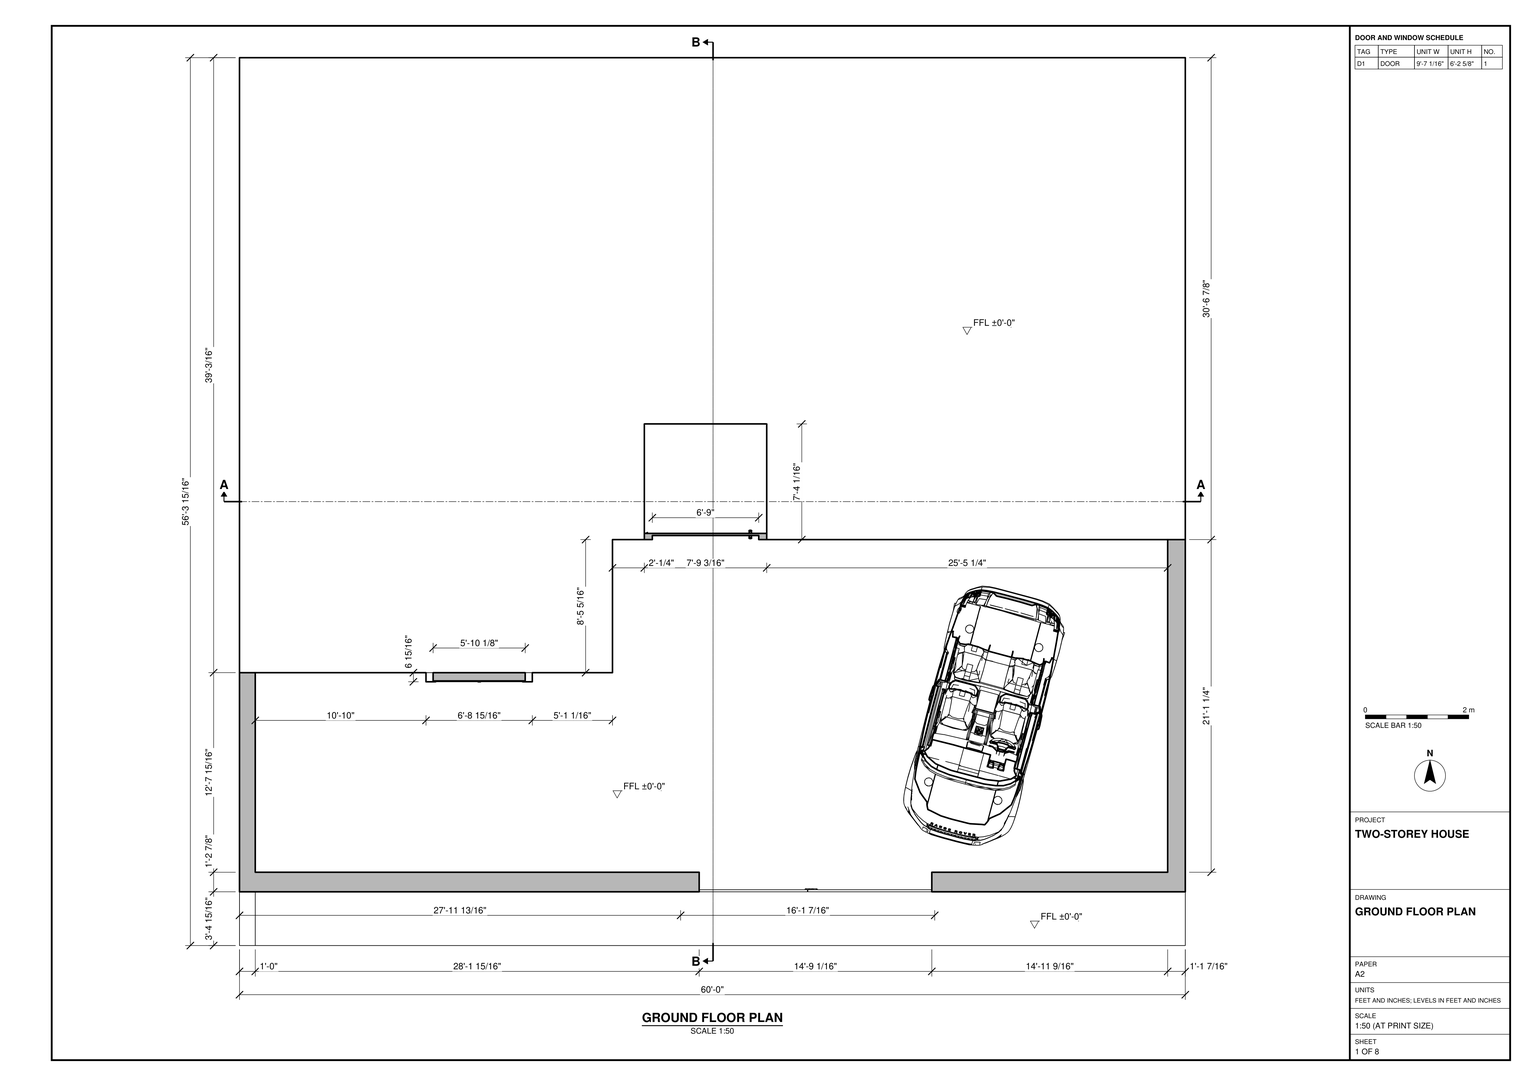
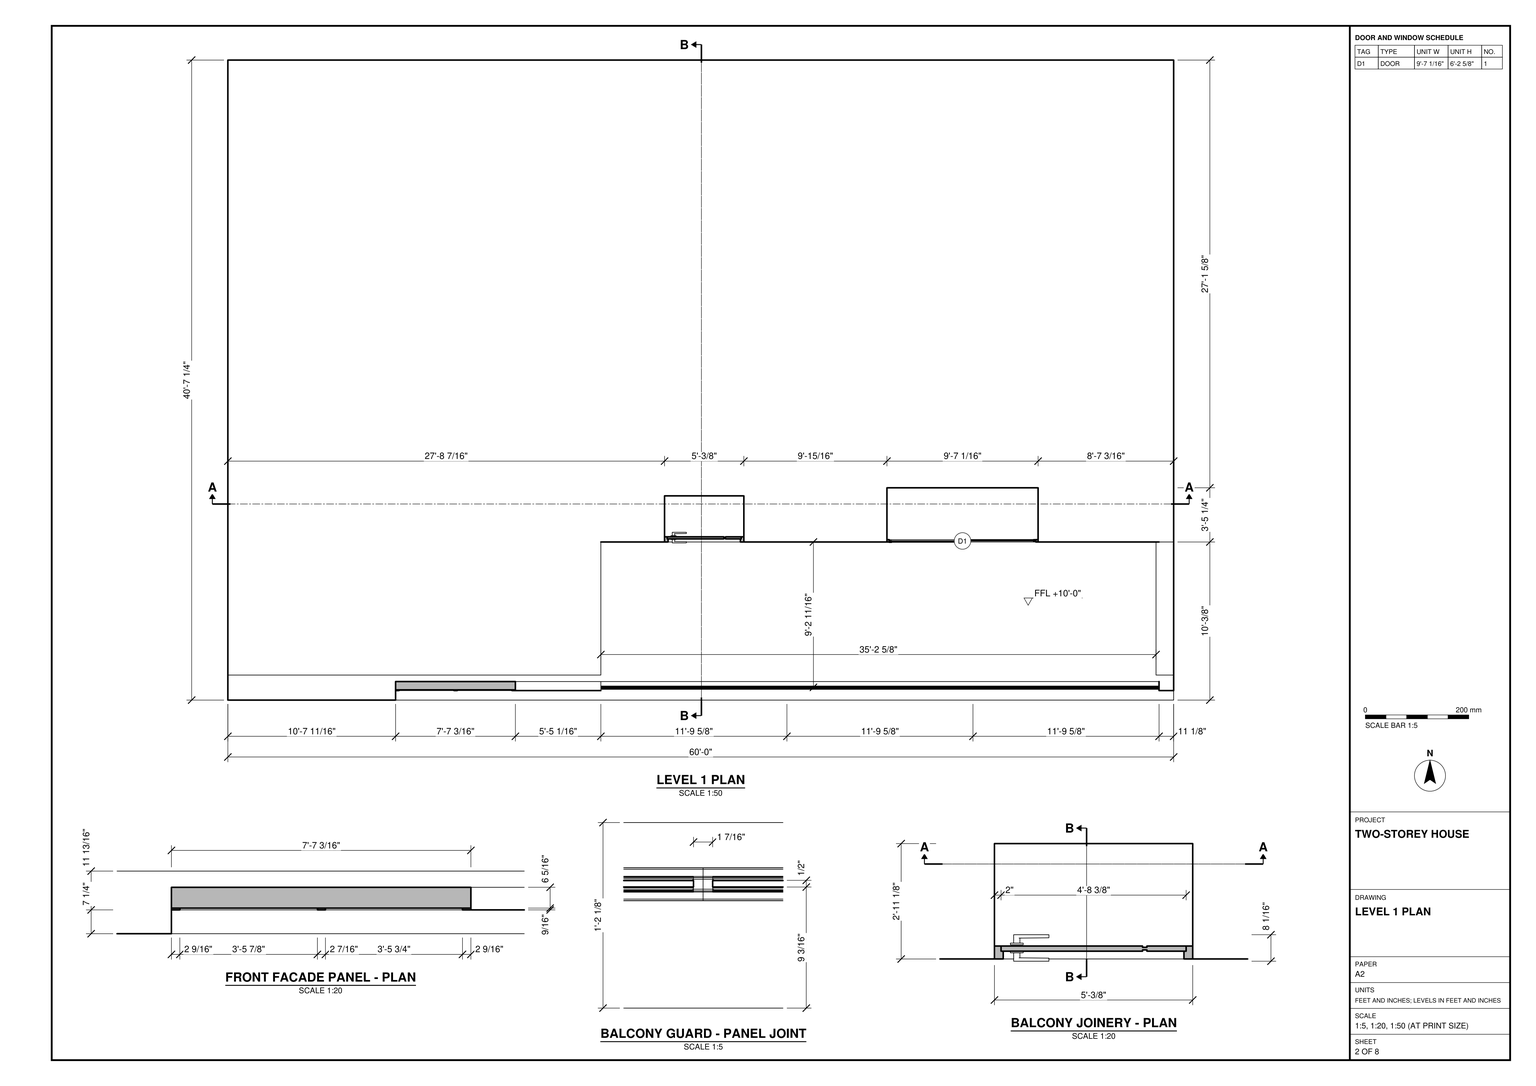
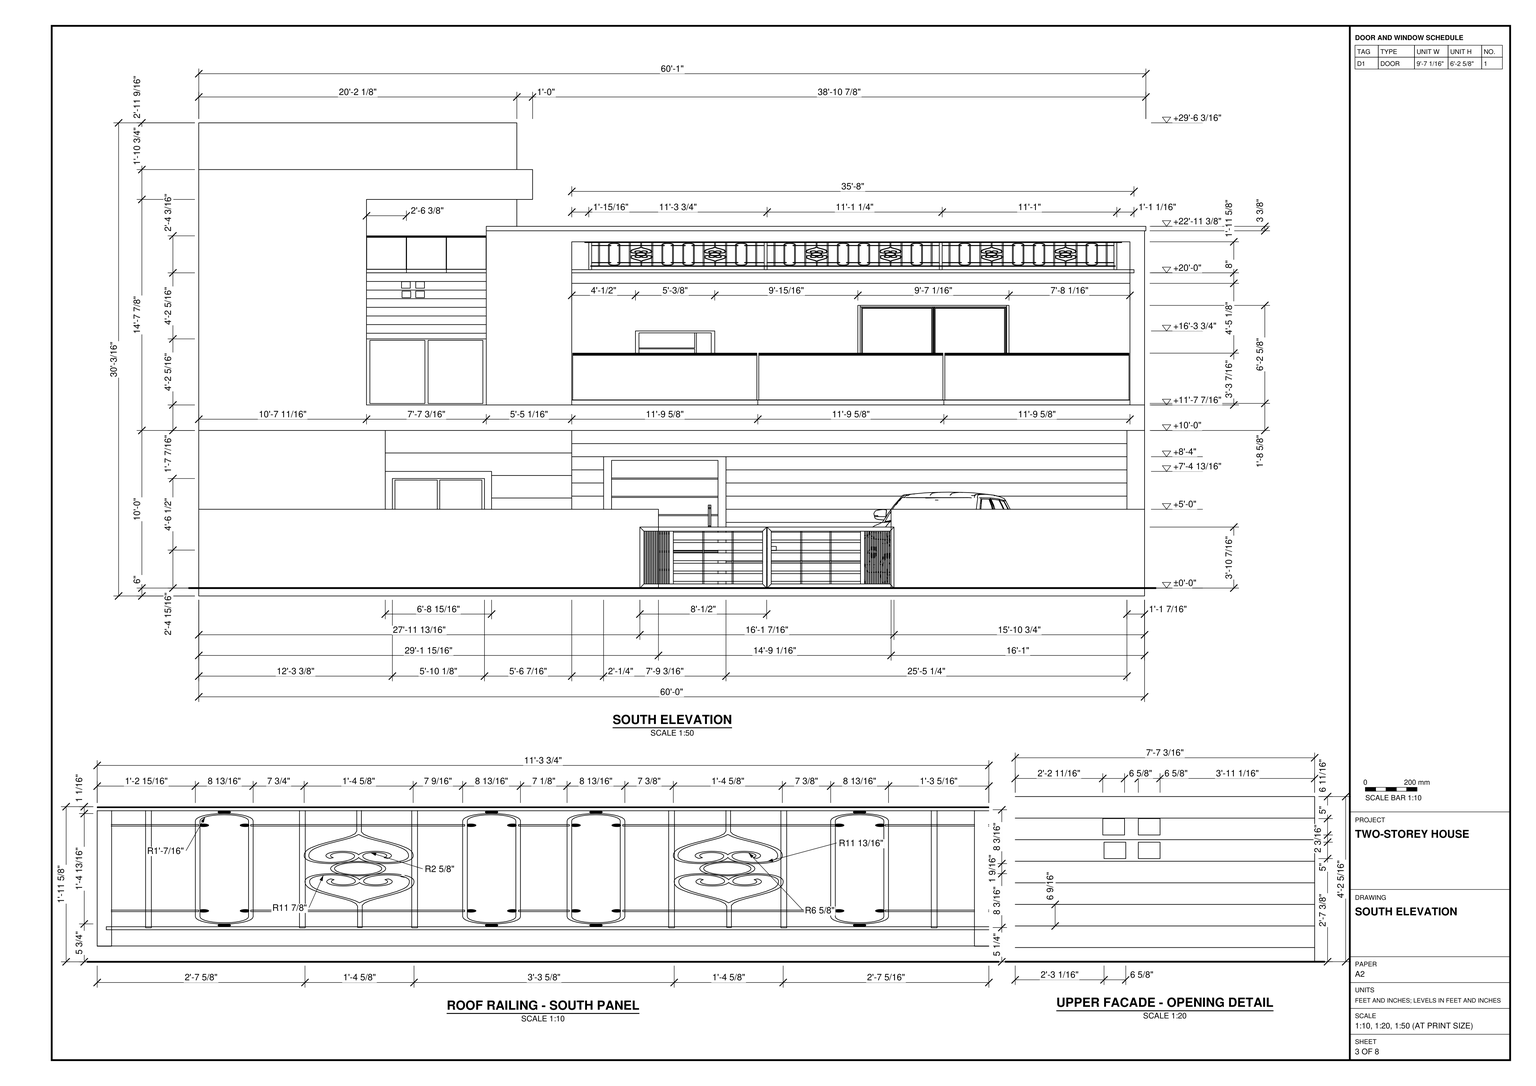
Build the two-storey house in SketchUp from task_files/diagram_01.pdf. Work in feet and inches. The overall model extents are 60'-1" along X, 56'-3 15/16" along Y and 30'-3/16" along Z. Set the ground floor at ±0'-0" and the upper floor at +10'-0".

Use the plans to place the stepped south wall: the left part projects into the forecourt, while the right part is set back behind the parking area. Model the floor slabs, exterior walls and low forecourt walls at the thicknesses drawn. Fit the double-leaf gate in the front wall and place the car on the right side of the forecourt.

Use the south elevation to set out the taller left volume, the flat roof slabs and the rectangular frame around the recessed upper balcony. Model the panel joints in the balcony guard, the wide door and the narrower joinery to its left. Follow the details for the banded facade panel and the repeating railing along the roof. Decor and loose items may be represented by any suitable library component.

Keep the walls, slabs and roof separate as groups or components, and group each furniture or joinery piece separately. Use components for repeated parts. Save one SketchUp model as output_files/two_storey_house_gated_forecourt_and_recessed_balcony.skp.

# SketchUp Ruby script. Lengths in inches.
U = 1.inch
M = Sketchup.active_model
def pt(a) = Geom::Point3d.new(a.map { |v| v * U })
def face(e, loops, mat)
  f = e.add_face(loops[0].map { |a| pt(a) })
  loops[1..].each { |l| e.add_face(l.map { |a| pt(a) }).erase! }
  f.material = f.back_material = mat if mat
  f
end
# faces: each face lists its corners as indices into pts; further lists are holes
def faces(e, pts, list, mat = nil) = list.each { |f| face(e, (f[0].is_a?(Array) ? f : [f]).map { |l| l.map { |i| pts[i] } }, mat) }
# xy, xz, yz: faces in a plane at the given z, y or x. An outline is a flat list of corners, or four numbers for a rectangle; further outlines are holes
def ring(l) = l.size == 4 ? [[l[0], l[1]], [l[2], l[1]], [l[2], l[3]], [l[0], l[3]]] : l.each_slice(2).to_a
def flat(e, list, mat, &to3) = list.each { |f| face(e, (f[0].is_a?(Array) ? f : [f]).map { |l| ring(l).map { |u, v| to3.(u, v) } }, mat) }
def xy(e, z, list, mat = nil) = flat(e, list, mat) { |x, y| [x, y, z] }
def xz(e, y, list, mat = nil) = flat(e, list, mat) { |x, z| [x, y, z] }
def yz(e, x, list, mat = nil) = flat(e, list, mat) { |y, z| [x, y, z] }
def lines(e, pts, list) = list.each { |a, b| e.add_line(pt(pts[a]), pt(pts[b])) }
# prism: a flat outline (further loops are holes) pulled along v
def prism(e, loops, v, mat = nil)
  f = face(e, loops, mat); d = Geom::Vector3d.new(v.map { |x| x * U })
  f.pushpull(f.normal.samedirection?(d) ? d.length : -d.length)
end
def box(e, o, s, mat = nil) = prism(e, [[o, [o[0] + s[0], o[1], o[2]], [o[0] + s[0], o[1] + s[1], o[2]], [o[0], o[1] + s[1], o[2]]]], [0, 0, s[2]], mat)
def at(x, y, z, deg = 0) = Geom::Transformation.translation(pt([x, y, z])) * Geom::Transformation.rotation(ORIGIN, Z_AXIS, deg.degrees)
def axes(o, x, y, z) = Geom::Transformation.new([*x, 0, *y, 0, *z, 0, *pt(o).to_a, 1])
def part(name) = M.definitions.add(name)
# library, detail: a bought-in or finely detailed component or shape, given as its bounding box
def library(name, o, s) = part(name).tap { |d| box(d.entities, o, s) }
def detail(e, o, s) = box(e.add_group.entities, o, s)
def put(e, d, t, mat = nil) = e.add_instance(d, t).tap { |i| i.material = mat if mat }
def group(e, t, mat = nil) = e.add_group.tap { |g| g.transformation = t; g.material = mat if mat }.entities
root = M.entities
M.materials.add("2 ").color = [128, 128, 128]
M.materials["2 "].alpha = 0.5
M.materials.add("Glass_Tinted_Gray").color = [0, 0, 0]
M.materials["Glass_Tinted_Gray"].alpha = 0.125
M.materials.add("Material60").color = [234, 198, 157]
M.materials.add("RDFGXVY 1").color = [35, 53, 69]
M.materials.add("[0086_MediumAquamarine]").color = [16, 35, 30]
M.materials.add("[0135_DarkGray]").color = [81, 81, 81]
M.materials.add("[0137_Black]").color = [0, 0, 0]
M.materials.add("[Color M00]").color = [255, 255, 255]
M.materials.add("[Color M04]").color = [142, 142, 142]
M.materials.add("[Mirror 02]").color = [229, 229, 229]
M.materials.add("[Slate Light Tile]").color = [54, 54, 54]
M.materials.add("[Terrazzo Light Blue]").color = [196, 214, 227]
M.materials.add("[Wood Veneer 01]").color = [120, 70, 37]
M.materials.add("[Wood Veneer 01]1").color = [119, 70, 35]
M.materials.add("ertg dfy 1").color = [92, 92, 92]
c1 = library("Glass Railings(black Handrails)",[-57.04,-132.55,0],[169.29,2.52,28.17])
c2 = part("Box01")
box(c2.entities,[-226.9,-4,10.92],[453.97,2,2],"RDFGXVY 1")
c3 = part("Box33")
box(c3.entities,[-243.2,-14.58,-10.36],[486.37,14.58,10.5],"ertg dfy 1")
c4 = part("Box45")
box(c4.entities,[-155.57,-3.5,79.72],[8.78,1,1],"RDFGXVY 1")
c5 = part("Box46")
box(c5.entities,[-201.91,-3.5,79.72],[37.02,1,1],"RDFGXVY 1")
c6 = part("Box48")
box(c6.entities,[-226.6,-3.5,79.72],[15.69,1,1],"RDFGXVY 1")
c7 = part("Box50")
box(c7.entities,[-220.1,-3.75,12.2],[1,1.5,78.43],"RDFGXVY 1")
c8 = part("Box51")
box(c8.entities,[-228.47,-4.25,0],[2.5,2.5,90.63],"RDFGXVY 1")
c9 = part("Donut06")
prism(c9.entities,[[[-187.98,-2.25,52.57],[-187.62,-2.25,53.58],[-187.05,-2.25,54.47],[-186.3125,-2.25,55.21],[-185.43,-2.25,55.77],[-184.42,-2.25,56.13],[-183.32,-2.25,56.26],[-182.23,-2.25,56.13],[-181.22,-2.25,55.77],[-180.34,-2.25,55.21],[-179.59,-2.25,54.47],[-179.03,-2.25,53.58],[-178.67,-2.25,52.57],[-178.54,-2.25,51.48],[-178.67,-2.25,50.38],[-179.03,-2.25,49.38],[-179.59,-2.25,48.49],[-180.34,-2.25,47.75],[-181.22,-2.25,47.18],[-182.23,-2.25,46.82],[-183.32,-2.25,46.7],[-184.42,-2.25,46.82],[-185.43,-2.25,47.18],[-186.3125,-2.25,47.75],[-187.05,-2.25,48.49],[-187.62,-2.25,49.38],[-187.98,-2.25,50.38],[-188.1,-2.25,51.48]],[[-186.52,-2.25,54.04],[-187.01,-2.25,53.28],[-187.32,-2.25,52.42],[-187.42,-2.25,51.48],[-187.32,-2.25,50.54],[-187.01,-2.25,49.68],[-186.52,-2.25,48.92],[-185.89,-2.25,48.28],[-185.125,-2.25,47.8],[-184.26,-2.25,47.49],[-183.32,-2.25,47.38],[-182.39,-2.25,47.49],[-181.52,-2.25,47.8],[-180.76,-2.25,48.28],[-180.125,-2.25,48.92],[-179.64,-2.25,49.68],[-179.33,-2.25,50.54],[-179.23,-2.25,51.48],[-179.33,-2.25,52.42],[-179.64,-2.25,53.28],[-180.125,-2.25,54.04],[-180.76,-2.25,54.68],[-181.52,-2.25,55.16],[-182.39,-2.25,55.47],[-183.32,-2.25,55.58],[-184.26,-2.25,55.47],[-185.125,-2.25,55.16],[-185.89,-2.25,54.68]]],[0,-1.5,0],"RDFGXVY 1")
c10 = library("Rectangl19",[-192.66,-3.75,54.81],[18.86,1.5,35.73])
c11 = part("Rectangl21")
prism(c11.entities,[[[-211.36,-2.25,18.49],[-211.49,-2.25,19.59],[-211.49,-2.25,83.23],[-211.36,-2.25,84.33],[-211,-2.25,85.34],[-210.43,-2.25,86.23],[-209.6875,-2.25,86.97],[-208.8,-2.25,87.54],[-207.79,-2.25,87.9],[-206.6875,-2.25,88.03],[-206.29,-2.25,88.03],[-205.1875,-2.25,87.9],[-204.18,-2.25,87.54],[-203.29,-2.25,86.97],[-202.54,-2.25,86.23],[-201.98,-2.25,85.34],[-201.62,-2.25,84.33],[-201.49,-2.25,83.23],[-201.49,-2.25,19.59],[-201.62,-2.25,18.49],[-201.98,-2.25,17.48],[-202.54,-2.25,16.59],[-203.29,-2.25,15.84],[-204.18,-2.25,15.28],[-205.1875,-2.25,14.92],[-206.29,-2.25,14.79],[-206.6875,-2.25,14.79],[-207.79,-2.25,14.92],[-208.8,-2.25,15.28],[-209.6875,-2.25,15.84],[-210.43,-2.25,16.59],[-211,-2.25,17.48]],[[-210.6875,-2.25,83.22],[-210.6875,-2.25,19.59],[-210.58,-2.25,18.68],[-210.28,-2.25,17.83],[-209.81,-2.25,17.09],[-209.1875,-2.25,16.47],[-208.44,-2.25,16],[-207.6,-2.25,15.7],[-206.68,-2.25,15.59],[-206.29,-2.25,15.59],[-205.375,-2.25,15.7],[-204.53,-2.25,16],[-203.79,-2.25,16.47],[-203.17,-2.25,17.09],[-202.7,-2.25,17.83],[-202.39,-2.25,18.68],[-202.29,-2.25,19.59],[-202.29,-2.25,83.22],[-202.39,-2.25,84.14],[-202.7,-2.25,84.98],[-203.17,-2.25,85.73],[-203.79,-2.25,86.35],[-204.53,-2.25,86.82],[-205.375,-2.25,87.12],[-206.29,-2.25,87.23],[-206.68,-2.25,87.23],[-207.6,-2.25,87.12],[-208.44,-2.25,86.82],[-209.1875,-2.25,86.35],[-209.81,-2.25,85.73],[-210.28,-2.25,84.98],[-210.58,-2.25,84.14]]],[0,-1.5,0],"RDFGXVY 1")
c12 = part("Rectangle0")
prism(c12.entities,[[[-231.96,-3.14,92.61],[-231.96,-1.96,92.53],[-231.96,-0.8125,92.24],[-231.96,0,91.89],[-231.96,0,89.89],[-231.96,-6,89.89],[-231.96,-6,91.89],[-231.96,-5.46,92.14],[-231.96,-4.32,92.48]]],[464.5,0,0],"RDFGXVY 1")
c13 = library("Sphere59",[-210.98,-3.9,79.34],[1.8,1.8,1.8])
c14 = library("Sphere66",[-207.6,-4.11,87.84],[2.22,2.22,2.22])
c15 = part("skp249")
put(c15.entities,c2,at(0,0,0))
put(c15.entities,c3,at(0,0,0))
put(c15.entities,c4,at(0,0,0))
put(c15.entities,c5,at(0,0,0))
put(c15.entities,c6,at(0,0,0))
put(c15.entities,c7,at(0,0,0))
put(c15.entities,c8,at(0,0,0))
put(c15.entities,c9,at(0,0,0))
put(c15.entities,c10,at(0,0,0))
put(c15.entities,c11,at(0,0,0))
put(c15.entities,c12,at(0,0,0))
put(c15.entities,c13,at(0,0,0))
put(c15.entities,c14,at(0,0,0))
put(c15.entities,c13,at(7.24,0,0))
put(c15.entities,c13,at(0,0,-56.78))
put(c15.entities,c13,at(7.24,0,-56.78))
put(c15.entities,c14,at(0,0,-75.08))
put(c15.entities,c6,at(0,0,-56.78))
put(c15.entities,c10,axes([0.14,0,102.9375],[1,0,0],[0,1,0],[0,0,-1]))
put(c15.entities,c5,at(0,0,-56.78))
put(c15.entities,c7,at(26.625,0,0))
put(c15.entities,c7,at(46.05,0,0))
put(c15.entities,c4,at(0,0,-56.78))
put(c15.entities,c14,at(46.25,0,0))
put(c15.entities,c13,at(46.25,0,0))
put(c15.entities,c13,at(53.48,0,0))
put(c15.entities,c13,at(53.48,0,-56.78))
put(c15.entities,c13,at(46.25,0,-56.78))
put(c15.entities,c14,at(46.25,0,-75.08))
put(c15.entities,c11,at(46.25,0,0))
put(c15.entities,c5,at(64.37,0,0))
put(c15.entities,c5,at(64.37,0,-56.78))
put(c15.entities,c11,at(64.3125,0,0))
put(c15.entities,c14,at(64.3125,0,-75.08))
put(c15.entities,c13,at(64.3125,0,-56.78))
put(c15.entities,c13,at(71.55,0,-56.78))
put(c15.entities,c13,at(71.55,0,0))
put(c15.entities,c13,at(64.3125,0,0))
put(c15.entities,c14,at(64.3125,0,0))
put(c15.entities,c7,at(90.5,0,0))
put(c15.entities,c7,at(109.92,0,0))
put(c15.entities,c10,at(63.875,0,0))
put(c15.entities,c10,axes([64.02,0,102.9375],[1,0,0],[0,1,0],[0,0,-1]))
put(c15.entities,c9,at(63.875,0,0))
put(c15.entities,c14,at(109.92,0,-75.08))
put(c15.entities,c13,at(117.16,0,0))
put(c15.entities,c13,at(109.92,0,0))
put(c15.entities,c14,at(109.92,0,0))
put(c15.entities,c13,at(109.92,0,-56.78))
put(c15.entities,c13,at(117.16,0,-56.78))
put(c15.entities,c11,at(109.92,0,0))
put(c15.entities,c7,at(135.9375,0,0))
put(c15.entities,c6,at(134.46,0,0))
put(c15.entities,c6,at(134.46,0,-56.78))
put(c15.entities,c8,at(151.78,0,0))
put(c15.entities,c7,at(151.78,0,0))
put(c15.entities,c6,at(151.78,0,0))
put(c15.entities,c6,at(151.78,0,-56.78))
put(c15.entities,c5,at(151.78,0,-56.78))
put(c15.entities,c7,at(178.4,0,0))
put(c15.entities,c7,at(197.83,0,0))
put(c15.entities,c14,at(151.78,0,-75.08))
put(c15.entities,c13,at(151.78,0,0))
put(c15.entities,c14,at(151.78,0,0))
put(c15.entities,c13,at(151.78,0,-56.78))
put(c15.entities,c13,at(159.01,0,-56.78))
put(c15.entities,c11,at(151.78,0,0))
put(c15.entities,c13,at(159.01,0,0))
put(c15.entities,c10,at(151.78,0,0))
put(c15.entities,c10,axes([151.92,0,102.9375],[1,0,0],[0,1,0],[0,0,-1]))
put(c15.entities,c9,at(151.78,0,0))
put(c15.entities,c5,at(151.78,0,0))
put(c15.entities,c4,at(151.78,0,0))
put(c15.entities,c4,at(151.78,0,-56.78))
put(c15.entities,c13,at(198.02,0,0))
put(c15.entities,c14,at(198.02,0,0))
put(c15.entities,c13,at(205.26,0,-56.78))
put(c15.entities,c11,at(198.02,0,0))
put(c15.entities,c13,at(205.26,0,0))
put(c15.entities,c13,at(198.02,0,-56.78))
put(c15.entities,c14,at(198.02,0,-75.08))
put(c15.entities,c5,at(216.14,0,0))
put(c15.entities,c5,at(216.14,0,-56.78))
put(c15.entities,c7,at(242.28,0,0))
put(c15.entities,c13,at(216.09,0,-56.78))
put(c15.entities,c14,at(216.09,0,-75.08))
put(c15.entities,c13,at(223.32,0,0))
put(c15.entities,c13,at(223.32,0,-56.78))
put(c15.entities,c14,at(216.09,0,0))
put(c15.entities,c11,at(216.09,0,0))
put(c15.entities,c13,at(216.09,0,0))
put(c15.entities,c7,at(261.69,0,0))
put(c15.entities,c10,at(215.65,0,0))
put(c15.entities,c10,axes([215.79,0,102.9375],[1,0,0],[0,1,0],[0,0,-1]))
put(c15.entities,c9,at(215.65,0,0))
put(c15.entities,c6,at(286.24,0,0))
put(c15.entities,c7,at(287.71,0,0))
put(c15.entities,c6,at(286.24,0,-56.78))
put(c15.entities,c7,at(303.21,0,0))
put(c15.entities,c13,at(268.93,0,0))
put(c15.entities,c14,at(261.69,0,-75.08))
put(c15.entities,c14,at(261.69,0,0))
put(c15.entities,c13,at(261.69,0,-56.78))
put(c15.entities,c13,at(268.93,0,-56.78))
put(c15.entities,c11,at(261.69,0,0))
put(c15.entities,c13,at(261.69,0,0))
put(c15.entities,c8,at(303.21,0,0))
put(c15.entities,c6,at(303.21,0,0))
put(c15.entities,c6,at(303.21,0,-56.78))
put(c15.entities,c7,at(329.83,0,0))
put(c15.entities,c7,at(349.26,0,0))
put(c15.entities,c5,at(303.21,0,0))
put(c15.entities,c5,at(303.21,0,-56.78))
put(c15.entities,c13,at(303.21,0,0))
put(c15.entities,c13,at(310.44,0,-56.78))
put(c15.entities,c14,at(303.21,0,-75.08))
put(c15.entities,c11,at(303.21,0,0))
put(c15.entities,c14,at(303.21,0,0))
put(c15.entities,c13,at(310.44,0,0))
put(c15.entities,c13,at(303.21,0,-56.78))
put(c15.entities,c10,at(303.21,0,0))
put(c15.entities,c9,at(303.21,0,0))
put(c15.entities,c10,axes([303.35,0,102.9375],[1,0,0],[0,1,0],[0,0,-1]))
put(c15.entities,c4,at(303.21,0,0))
put(c15.entities,c4,at(303.21,0,-56.78))
put(c15.entities,c14,at(349.45,0,0))
put(c15.entities,c13,at(349.45,0,0))
put(c15.entities,c11,at(349.45,0,0))
put(c15.entities,c14,at(349.45,0,-75.08))
put(c15.entities,c13,at(356.69,0,0))
put(c15.entities,c13,at(356.69,0,-56.78))
put(c15.entities,c13,at(349.45,0,-56.78))
put(c15.entities,c5,at(367.57,0,0))
put(c15.entities,c5,at(367.57,0,-56.78))
put(c15.entities,c14,at(367.52,0,0))
put(c15.entities,c13,at(374.76,0,0))
put(c15.entities,c14,at(367.52,0,-75.08))
put(c15.entities,c13,at(374.76,0,-56.78))
put(c15.entities,c11,at(367.52,0,0))
put(c15.entities,c13,at(367.52,0,0))
put(c15.entities,c13,at(367.52,0,-56.78))
put(c15.entities,c7,at(393.71,0,0))
put(c15.entities,c7,at(413.125,0,0))
put(c15.entities,c10,at(367.08,0,0))
put(c15.entities,c10,axes([367.22,0,102.9375],[1,0,0],[0,1,0],[0,0,-1]))
put(c15.entities,c9,at(367.08,0,0))
put(c15.entities,c6,at(437.67,0,0))
put(c15.entities,c6,at(437.67,0,-56.78))
put(c15.entities,c7,at(439.14,0,0))
put(c15.entities,c8,at(454.3125,0,0))
put(c15.entities,c13,at(420.36,0,0))
put(c15.entities,c13,at(420.36,0,-56.78))
put(c15.entities,c14,at(413.125,0,-75.08))
put(c15.entities,c13,at(413.125,0,-56.78))
put(c15.entities,c11,at(413.125,0,0))
put(c15.entities,c14,at(413.125,0,0))
put(c15.entities,c13,at(413.125,0,0))
c16 = part("Railing1")
put(c16.entities,c15,at(243.2,14.58,10.36))
c17 = library("PINTU 6 YA",[0,-0.6875,0],[35.83,8.07,80.71])
c18 = part("PENTEK_RP Fineline 50S_Sliding_DoorCase_E1")
box(c18.entities,[0,0,0],[1.51,3.66,99.27],"[0135_DarkGray]")
c19 = part("PENTEK_RP Fineline 50S_SlidingDooe_Case_E2")
box(c19.entities,[0,0,0],[96.25,3.66,1.51],"[0135_DarkGray]")
c20 = part("pentek_RP Fineline 50S_SlidingDoor_Case")
put(c20.entities,c18,at(97.76,0,0))
put(c20.entities,c19,at(1.51,0,0))
put(c20.entities,c18,at(0,0,0))
put(c20.entities,c19,at(1.51,0,97.76))
c21 = part("PENTEK_RP Fineline 50S_SlidingDoor_GlazingBead_2")
box(c21.entities,[0,0,0],[0.56,0.59,94.39],"[0135_DarkGray]")
c22 = part("PENTEK_RP Fineline 50S_SlidingDoor_Glass")
box(c22.entities,[0,0,0],[46.58,0.16,94.39],"Glass_Tinted_Gray")
c23 = part("PENTEK_RP Fineline 50S_SlidingDoor_GlazingBead")
box(c23.entities,[0,0,0],[45.47,0.59,0.56],"[0135_DarkGray]")
c24 = part("PENTEK_RP Fineline 50S_SlidingDoor_Leaf_E1")
xy(c24.entities,0,[[0,0,0.93,1.97],[0.93,1.57,1.49,1.97]],"[0135_DarkGray]")
xy(c24.entities,96.25,[[0,0,0.93,0,0.93,1.57,1.49,1.57,1.49,1.97,0,1.97]],"[0135_DarkGray]")
xz(c24.entities,0,[[0,0,0.93,96.25]],"[0135_DarkGray]")
xz(c24.entities,1.57,[[0.93,0,1.49,95.32],[0.93,95.32,1.49,96.25]],"[0135_DarkGray]")
xz(c24.entities,1.97,[[0,0,1.49,96.25]],"[0135_DarkGray]")
yz(c24.entities,0,[[0,0,1.97,96.25]],"[0135_DarkGray]")
yz(c24.entities,0.93,[[0,0,1.57,0.93],[0,0.93,1.57,95.32],[0,95.32,1.57,96.25]],"[0135_DarkGray]")
yz(c24.entities,1.49,[[1.57,0,1.97,95.32],[1.57,95.32,1.97,96.25]],"[0135_DarkGray]")
c25 = part("PENTEK_RP Fineline 50S_SlidingDoor_Leaf_E2")
xy(c25.entities,0,[[0,0,0,1.57,0.56,1.57,0.56,1.97,46.02,1.97,46.02,1.57,46.58,1.57,46.58,0]],"[0135_DarkGray]")
xy(c25.entities,0.93,[[0,0,46.58,1.57]],"[0135_DarkGray]")
xy(c25.entities,1.49,[[0.56,1.57,46.02,1.97]],"[0135_DarkGray]")
xz(c25.entities,0,[[0,0,46.58,0.93]],"[0135_DarkGray]")
xz(c25.entities,1.57,[[0,0,0.56,0.93],[46.02,0,46.58,0.93],[0.56,0.93,46.02,1.49]],"[0135_DarkGray]")
xz(c25.entities,1.97,[[0.56,0,46.02,1.49]],"[0135_DarkGray]")
yz(c25.entities,0,[[0,0,1.57,0.93]],"[0135_DarkGray]")
yz(c25.entities,0.56,[[1.57,0,1.97,0.93],[1.57,0.93,1.97,1.49]],"[0135_DarkGray]")
yz(c25.entities,46.02,[[1.57,0,1.97,0.93],[1.57,0.93,1.97,1.49]],"[0135_DarkGray]")
yz(c25.entities,46.58,[[0,0,1.57,0.93]],"[0135_DarkGray]")
c26 = part("PENTEK_RP Fineline S_SlidingDoor_Leaf1")
put(c26.entities,c21,at(0.93,0,0.93))
put(c26.entities,c21,at(46.96,0,0.93))
put(c26.entities,c22,at(1.49,1.42,0.93))
put(c26.entities,c23,at(1.49,0,0.93))
put(c26.entities,c22,at(1.49,0.59,0.93),"[Terrazzo Light Blue]")
put(c26.entities,c24,at(0,0,0))
put(c26.entities,c24,axes([48.44,0,0],[-1,0,0],[0,1,0],[0,0,1]))
put(c26.entities,c25,axes([0.93,0,96.25],[1,0,0],[0,1,0],[0,0,-1]))
put(c26.entities,c25,at(0.93,0,0))
put(c26.entities,c23,at(1.49,0,94.77))
c27 = part("PENTEK_RP Fineline 50S_SlidingDoor_Leaf2")
put(c27.entities,c22,at(1.49,1.42,0.93))
put(c27.entities,c23,at(1.49,0,94.77))
put(c27.entities,c21,at(46.96,0,0.93))
put(c27.entities,c22,at(1.49,0.59,0.93),"[Mirror 02]")
put(c27.entities,c21,at(0.93,0,0.93))
put(c27.entities,c24,at(0,0,0))
put(c27.entities,c24,axes([48.44,0,0],[-1,0,0],[0,1,0],[0,0,1]))
put(c27.entities,c23,at(1.49,0,0.93))
put(c27.entities,c25,axes([0.93,0,96.25],[1,0,0],[0,1,0],[0,0,-1]))
put(c27.entities,c25,at(0.93,0,0))
c28 = part("PENTEK - Slimmest Steel Sliding Door / Window\#1")
put(c28.entities,c20,at(0,-1.88,-0.09))
put(c28.entities,c26,at(1.51,-2.27,1.42))
put(c28.entities,c27,at(49.32,-0.3,1.42))
c29 = part("Group\#8")
xy(c29.entities,0,[[0.39,1.57,0.29,1.59,0.2,1.63,0.12,1.69,0.05,1.77,0.01,1.87,0,1.97,0.01,2.07,0.05,2.17,0.12,2.25,0.2,2.31,0.29,2.35,0.39,2.36,0.5,2.35,0.59,2.31,0.67,2.25,0.73,2.17,0.77,2.07,0.79,1.97,0.77,1.87,0.73,1.77,0.67,1.69,0.59,1.63,0.5,1.59],[0.39,13.39,0.29,13.4,0.2,13.4375,0.12,13.5,0.05,13.58,0.01,13.68,0,13.78,0.01,13.88,0.05,13.98,0.12,14.06,0.2,14.12,0.29,14.16,0.39,14.17,0.5,14.16,0.59,14.12,0.67,14.06,0.73,13.98,0.77,13.88,0.79,13.78,0.77,13.68,0.73,13.58,0.67,13.5,0.59,13.4375,0.5,13.4]])
xy(c29.entities,1.97,[[0.39,1.57,0.39,2.36,0.29,2.35,0.2,2.31,0.12,2.25,0.05,2.17,0.01,2.07,0,1.97,0.01,1.87,0.05,1.77,0.12,1.69,0.2,1.63,0.29,1.59],[0.39,1.57,0.5,1.59,0.59,1.63,0.67,1.69,0.73,1.77,0.77,1.87,0.79,1.97,0.77,2.07,0.73,2.17,0.67,2.25,0.59,2.31,0.5,2.35,0.39,2.36],[0.39,13.39,0.39,14.17,0.29,14.16,0.2,14.12,0.12,14.06,0.05,13.98,0.01,13.88,0,13.78,0.01,13.68,0.05,13.58,0.12,13.5,0.2,13.4375,0.29,13.4],[0.39,13.39,0.5,13.4,0.59,13.4375,0.67,13.5,0.73,13.58,0.77,13.68,0.79,13.78,0.77,13.88,0.73,13.98,0.67,14.06,0.59,14.12,0.5,14.16,0.39,14.17]])
xz(c29.entities,0,[[0.39,1.57,0.5,1.59,0.59,1.63,0.67,1.69,0.73,1.77,0.77,1.87,0.79,1.97,0.77,2.07,0.73,2.17,0.67,2.25,0.59,2.31,0.5,2.35,0.39,2.36,0.29,2.35,0.2,2.31,0.12,2.25,0.05,2.17,0.01,2.07,0,1.97,0.01,1.87,0.05,1.77,0.12,1.69,0.2,1.63,0.29,1.59]])
xz(c29.entities,15.75,[[0.39,1.57,0.29,1.59,0.2,1.63,0.12,1.69,0.05,1.77,0.01,1.87,0,1.97,0.01,2.07,0.05,2.17,0.12,2.25,0.2,2.31,0.29,2.35,0.39,2.36,0.5,2.35,0.59,2.31,0.67,2.25,0.73,2.17,0.77,2.07,0.79,1.97,0.77,1.87,0.73,1.77,0.67,1.69,0.59,1.63,0.5,1.59]])
p = [[0.12,1.69,0],[0.2,1.63,0],[0.2,1.63,1.63],[0.2,1.63,1.97],[0.12,1.69,1.97],[0.12,1.69,1.69],
  [0.29,1.59,0],[0.29,1.59,1.59],[0.29,1.59,1.97],[0.39,1.57,0],[0.39,1.57,1.57],[0.39,1.57,1.97],
  [0.5,1.59,0],[0.5,1.59,1.59],[0.5,1.59,1.97],[0.59,1.63,0],[0.59,1.63,1.63],[0.59,1.63,1.97],
  [0.67,1.69,0],[0.67,1.69,1.69],[0.67,1.69,1.97],[0.05,1.77,0],[0.05,1.77,1.97],[0.05,1.77,1.77],
  [0.73,1.77,0],[0.73,1.77,1.77],[0.73,1.77,1.97],[0.01,1.87,0],[0.01,1.87,1.97],[0.01,1.87,1.87],
  [0.77,1.87,0],[0.77,1.87,1.87],[0.77,1.87,1.97],[0,1.97,0],[0,1.97,1.97],[0.79,1.97,0],
  [0.79,1.97,1.97],[0.01,2.07,0],[0.01,2.07,1.97],[0.01,2.07,1.87],[0.77,2.07,0],[0.77,2.07,1.87],
  [0.77,2.07,1.97],[0.05,2.17,0],[0.05,2.17,1.97],[0.05,2.17,1.77],[0.73,2.17,0],[0.73,2.17,1.77],
  [0.73,2.17,1.97],[0.12,2.25,0],[0.12,2.25,1.97],[0.12,2.25,1.69],[0.2,2.31,0],[0.2,2.31,1.97],
  [0.2,2.31,1.63],[0.67,2.25,0],[0.59,2.31,0],[0.59,2.31,1.63],[0.59,2.31,1.97],[0.67,2.25,1.97],
  [0.67,2.25,1.69],[0.29,2.35,0],[0.29,2.35,1.97],[0.29,2.35,1.59],[0.39,2.36,0],[0.39,2.36,1.97],
  [0.39,2.36,1.57],[0.5,2.35,0],[0.5,2.35,1.97],[0.5,2.35,1.59],[0.12,13.5,0],[0.2,13.4375,0],
  [0.2,13.4375,1.63],[0.2,13.4375,1.97],[0.12,13.5,1.97],[0.12,13.5,1.69],[0.29,13.4,0],[0.29,13.4,1.59],
  [0.29,13.4,1.97],[0.39,13.39,0],[0.39,13.39,1.57],[0.39,13.39,1.97],[0.5,13.4,0],[0.5,13.4,1.59],
  [0.5,13.4,1.97],[0.59,13.4375,0],[0.59,13.4375,1.63],[0.59,13.4375,1.97],[0.67,13.5,0],[0.67,13.5,1.69],
  [0.67,13.5,1.97],[0.05,13.58,0],[0.05,13.58,1.97],[0.05,13.58,1.77],[0.73,13.58,0],[0.73,13.58,1.77],
  [0.73,13.58,1.97],[0.01,13.68,0],[0.01,13.68,1.97],[0.01,13.68,1.87],[0.77,13.68,0],[0.77,13.68,1.87],
  [0.77,13.68,1.97],[0,13.78,0],[0,13.78,1.97],[0.79,13.78,0],[0.79,13.78,1.97],[0.01,13.88,0],
  [0.01,13.88,1.97],[0.01,13.88,1.87],[0.77,13.88,0],[0.77,13.88,1.87],[0.77,13.88,1.97],[0.05,13.98,0],
  [0.05,13.98,1.97],[0.05,13.98,1.77],[0.73,13.98,0],[0.73,13.98,1.77],[0.73,13.98,1.97],[0.12,14.06,0],
  [0.12,14.06,1.97],[0.12,14.06,1.69],[0.67,14.06,0],[0.67,14.06,1.69],[0.67,14.06,1.97],[0.2,14.12,0],
  [0.2,14.12,1.97],[0.2,14.12,1.63],[0.29,14.16,0],[0.29,14.16,1.97],[0.29,14.16,1.59],[0.59,14.12,0],
  [0.5,14.16,0],[0.5,14.16,1.59],[0.5,14.16,1.97],[0.59,14.12,1.97],[0.59,14.12,1.63],[0.39,14.17,0],
  [0.39,14.17,1.97],[0.39,14.17,1.57],[0.12,15.75,1.69],[0.2,15.75,1.63],[0.2,0,1.63],[0.12,0,1.69],
  [0.29,15.75,1.59],[0.29,0,1.59],[0.39,15.75,1.57],[0.39,13.78,1.57],[0.39,1.97,1.57],[0.39,0,1.57],
  [0.5,15.75,1.59],[0.5,0,1.59],[0.59,15.75,1.63],[0.59,0,1.63],[0.67,15.75,1.69],[0.67,0,1.69],
  [0.05,15.75,1.77],[0.05,0,1.77],[0.73,15.75,1.77],[0.73,0,1.77],[0.01,15.75,1.87],[0.01,0,1.87],
  [0.77,15.75,1.87],[0.77,0,1.87],[0,15.75,1.97],[0,0,1.97],[0.79,15.75,1.97],[0.79,0,1.97],
  [0.01,15.75,2.07],[0.01,0,2.07],[0.77,15.75,2.07],[0.77,0,2.07],[0.05,15.75,2.17],[0.05,0,2.17],
  [0.73,15.75,2.17],[0.73,0,2.17],[0.12,15.75,2.25],[0.12,0,2.25],[0.2,15.75,2.31],[0.2,0,2.31],
  [0.67,15.75,2.25],[0.59,15.75,2.31],[0.59,0,2.31],[0.67,0,2.25],[0.29,15.75,2.35],[0.29,0,2.35],
  [0.39,15.75,2.36],[0.39,0,2.36],[0.5,15.75,2.35],[0.5,0,2.35],[0.39,1.97,1.97],[0.39,13.78,0],
  [0.39,1.97,0],[0.39,13.78,1.97],[0.39,0,1.97],[0.39,15.75,1.97]]
faces(c29.entities,p,[[0,1,2,3,4,5],[1,6,7,8,3,2],[6,9,10,11,8,7],[9,12,13,14,11,10],[12,15,16,17,14,13],[15,18,19,20,17,16],[21,0,5,4,22,23],[18,24,25,26,20,19],
  [27,21,23,22,28,29],[24,30,31,32,26,25],[33,27,29,28,34],[30,35,36,32,31],[37,33,34,38,39],[35,40,41,42,36],[43,37,39,38,44,45],[40,46,47,48,42,41],
  [49,43,45,44,50,51],[52,49,51,50,53,54],[55,56,57,58,59,60],[46,55,60,59,48,47],[61,52,54,53,62,63],[64,61,63,62,65,66],[67,64,66,65,68,69],[56,67,69,68,58,57],
  [70,71,72,73,74,75],[71,76,77,78,73,72],[76,79,80,81,78,77],[79,82,83,84,81,80],[82,85,86,87,84,83],[85,88,89,90,87,86],[91,70,75,74,92,93],[88,94,95,96,90,89],
  [97,91,93,92,98,99],[94,100,101,102,96,95],[103,97,99,98,104],[100,105,106,102,101],[107,103,104,108,109],[105,110,111,112,106],[113,107,109,108,114,115],[110,116,117,118,112,111],
  [119,113,115,114,120,121],[116,122,123,124,118,117],[125,119,121,120,126,127],[128,125,127,126,129,130],[131,132,133,134,135,136],[122,131,136,135,124,123],[137,128,130,129,138,139],[132,137,139,138,134,133],
  [140,141,127,72,54,2,142,143,5,51,75,121],[141,144,130,77,63,7,145,142,2,54,72,127],[144,146,139,147,80,66,148,10,149,145,7,63,77,130],[146,150,133,83,69,13,151,149,10,148,66,80,147,139],[150,152,136,86,57,16,153,151,13,69,83,133],[152,154,123,89,60,19,155,153,16,57,86,136],[156,140,121,75,51,5,143,157,23,45,93,115],[154,158,117,95,47,25,159,155,19,60,89,123],
  [160,156,115,93,45,23,157,161,29,39,99,109],[158,162,111,101,41,31,163,159,25,47,95,117],[164,160,109,99,39,29,161,165,34,104],[162,166,106,36,167,163,31,41,101,111],[168,164,104,34,165,169],[166,170,171,167,36,106],[172,168,169,173],[170,174,175,171],
  [176,172,173,177],[178,176,177,179],[180,181,182,183],[174,180,183,175],[184,178,179,185],[186,184,185,187],[188,186,187,189],[181,188,189,182]])
lines(c29.entities,p,[[190,148],[191,147],[148,192],[147,193],[11,194],[138,195],[81,65]])
c30 = part("3+80")
p = [[0,0,0],[1,0,0],[1,1,0]]
lines(c30.entities,p,[[0,1],[1,2],[2,0]])
g1 = group(c30.entities,at(0,0.01,-0.01))
g2 = group(g1,at(0,0,0))
xy(g2,0.01,[[0,-4.72,2.36,0],[33.86,-4.72,36.22,0],[2.36,-1.57,33.86,0]])
xy(g2,11.42,[[2.36,-1.97,33.86,-1.57]],"[Color M04]")
xy(g2,12.2,[[2.36,-1.97,33.86,-1.57]],"[Color M04]")
xy(g2,23.23,[[2.36,-1.97,33.86,-1.57]],"[Color M04]")
xy(g2,24.02,[[2.36,-1.97,33.86,-1.57]],"[Color M04]")
xy(g2,35.04,[[2.36,-1.97,33.86,-1.57]],"[Color M04]")
xy(g2,35.83,[[2.36,-1.97,33.86,-1.57]],"[Color M04]")
xy(g2,46.85,[[2.36,-2.36,33.86,-1.57]],"[Color M04]")
xy(g2,47.64,[[2.36,-2.36,33.86,-1.57]],"[Color M04]")
xy(g2,58.66,[[2.36,-2.36,33.86,-1.57]],"[Color M04]")
xy(g2,59.45,[[2.36,-2.36,33.86,-1.57]],"[Color M04]")
xy(g2,70.47,[[2.36,-2.36,33.86,-1.57]],"[Color M04]")
xy(g2,71.26,[[2.36,-2.36,33.86,-1.57]],"[Color M04]")
xy(g2,82.68,[[2.36,-4.72,33.86,-1.57]],"[Wood Veneer 01]1")
xy(g2,85.04,[[0,-4.72,36.22,0]],"[Wood Veneer 01]1")
xz(g2,-4.72,[[0,0.01,0,85.04,36.22,85.04,36.22,0.01,33.86,0.01,33.86,82.68,2.36,82.68,2.36,0.01]],"[Wood Veneer 01]1")
xz(g2,-2.36,[[2.36,46.85,33.86,47.64],[2.36,58.66,33.86,59.45],[2.36,70.47,33.86,71.26]],"[Color M04]")
xz(g2,-1.97,[[2.36,11.42,33.86,12.2],[2.36,23.23,33.86,24.02],[2.36,35.04,33.86,35.83]],"[Color M04]")
xz(g2,-1.57,[[2.36,0.01,33.86,11.42],[2.36,12.2,33.86,23.23],[2.36,24.02,33.86,35.04],[2.36,35.83,33.86,46.85],[2.36,47.64,33.86,58.66],
  [2.36,59.45,33.86,70.47],[2.36,71.26,33.86,82.68]],"[Wood Veneer 01]1")
xz(g2,0,[[0,0.01,2.36,0.01,2.36,82.68,33.86,82.68,33.86,0.01,36.22,0.01,36.22,85.04,0,85.04],[2.36,0.01,33.86,82.68]],"[Wood Veneer 01]1")
yz(g2,0,[[-4.72,0.01,0,85.04]],"[Wood Veneer 01]1")
yz(g2,2.36,[[-4.72,0.01,-4.72,82.68,-1.57,82.68,-1.57,71.26,-2.36,71.26,-2.36,70.47,-1.57,70.47,-1.57,59.45,-2.36,59.45,-2.36,58.66,-1.57,58.66,-1.57,47.64,-2.36,47.64,-2.36,46.85,-1.57,46.85,-1.57,35.83,-1.97,35.83,-1.97,35.04,-1.57,35.04,-1.57,24.02,-1.97,24.02,-1.97,23.23,-1.57,23.23,-1.57,12.2,-1.97,12.2,-1.97,11.42,-1.57,11.42,-1.57,0.01]],"[Wood Veneer 01]1")
yz(g2,33.86,[[-4.72,0.01,-1.57,0.01,-1.57,11.42,-1.97,11.42,-1.97,12.2,-1.57,12.2,-1.57,23.23,-1.97,23.23,-1.97,24.02,-1.57,24.02,-1.57,35.04,-1.97,35.04,-1.97,35.83,-1.57,35.83,-1.57,46.85,-2.36,46.85,-2.36,47.64,-1.57,47.64,-1.57,58.66,-2.36,58.66,-2.36,59.45,-1.57,59.45,-1.57,70.47,-2.36,70.47,-2.36,71.26,-1.57,71.26,-1.57,82.68,-4.72,82.68]],"[Wood Veneer 01]1")
yz(g2,36.22,[[-4.72,0.01,0,85.04]],"[Wood Veneer 01]1")
p = [[0,0,0],[0,0,0.01]]
lines(g2,p,[[0,1]])
put(g1,c29,axes([30.98,0,38.01],[1,0,0],[0,0,1],[0,1,0]),"[Color M04]")
put(g1,c29,axes([30.98,-1.57,38.01],[1,0,0],[0,0,1],[0,-1,0]),"[Color M04]")
c31 = part("WindowDoubleBlack")
xy(c31.entities,0,[[0,0,96.0625,1.57]],"[0137_Black]")
xy(c31.entities,2.71,[[2.71,0,46.85,1.57],[49.41,0,93.35,1.57]],"[0137_Black]")
xy(c31.entities,122.09,[[2.71,0,46.85,1.57],[49.41,0,50,1.57],[50,0,93.35,1.57]],"[0137_Black]")
xy(c31.entities,124.8,[[0,0,96.0625,1.57]],"[0137_Black]")
xz(c31.entities,0,[[[0,0,96.0625,124.8],[2.71,2.71,46.85,122.09],[49.41,2.71,93.35,122.09]]],"[0137_Black]")
xz(c31.entities,1.57,[[2.71,2.71,46.85,122.09],[49.41,2.71,93.35,122.09]],"2 ")
xz(c31.entities,1.57,[[[0,0,96.0625,124.8],[2.71,2.71,46.85,122.09],[49.41,2.71,93.35,122.09]]],"[0137_Black]")
yz(c31.entities,0,[[0,0,1.57,124.8]],"[0137_Black]")
yz(c31.entities,2.71,[[0,2.71,1.57,122.09]],"[0137_Black]")
yz(c31.entities,46.85,[[0,2.71,1.57,122.09]],"[0137_Black]")
yz(c31.entities,49.41,[[0,2.71,1.57,122.09]],"[0137_Black]")
yz(c31.entities,93.35,[[0,2.71,1.57,122.09]],"[0137_Black]")
yz(c31.entities,96.0625,[[0,0,1.57,124.8]],"[0137_Black]")
c32 = library("Untitled",[131.66,19.68,0],[2.41,197.25,46.46])
c33 = library("RANGE ROVER",[-63.71,-35.21,42.76],[182.88,182.88,64.08])
c34 = part("Bilal architect uae abu dhabi ")
put(c34.entities,c33,axes([104.22,-10.75,-48.75],[0.98727,0.57,0],[-0.57,0.98727,0],[0,0,1.14]),"Material60")
xy(root,-6,[[0,0,720,675.9375]])
xy(root,0,[[0,0,12,40.91],[12,0,720,0,720,40.91,527.02,40.91,527.02,55.81,706.58,55.81,706.58,309.0625,401.36,309.0625,401.36,397.125,308.19,397.125,308.19,309.0625,283.94,309.0625,283.94,207.75,12,207.75,12,55.81,349.9375,55.81,349.9375,40.91,12,40.91],[0,40.91,0,207.75,12,207.75,12,55.81,349.9375,55.81,349.9375,40.91],[0,207.75,283.94,207.75,283.94,309.0625,308.19,309.0625,308.19,397.125,401.36,397.125,401.36,309.0625,720,309.0625,720,675.9375,0,675.9375]])
xy(root,23.51,[[141.97,200.8125,222.91,207.75]])
xy(root,28.92,[[147.38,200.8125,217.5,207.75]])
xy(root,60,[[0,40.91,349.9375,40.91,349.9375,55.81,12,55.81,12,207.75,0,207.75],[527.02,40.91,720,40.91,720,207.75,706.58,207.75,706.58,55.81,527.02,55.81]])
xy(root,83.41,[[147.38,200.8125,217.5,207.75]])
xy(root,88.82,[[141.97,200.8125,222.91,207.75]])
xy(root,100,[[308.19,309.0625,401.36,397.125]])
xy(root,120,[[0,188.6875,720,188.6875,720,207.75,706.58,207.75,706.58,309.0625,283.94,309.0625,283.94,207.75,0,207.75],[332.4375,309.0625,392.8125,344.1875]])
xy(root,139.42,[[218.88,195.9375,283.94,202.8125]])
xy(root,139.42,[[127.6875,188.6875,720,188.6875,720,195.9375,708.875,195.9375,708.875,202.8125,283.94,202.8125,283.94,195.9375,218.88,195.9375,218.88,202.8125,127.6875,202.8125]],"[Wood Veneer 01]")
xy(root,140.6,[[501.74,309.0625,616.8,350.3125]])
xy(root,189.71,[[127.6875,182,218.88,202.8125]],"[0086_MediumAquamarine]")
xy(root,194.02,[[127.6875,182,218.88,202.8125]],"[0086_MediumAquamarine]")
xy(root,195.75,[[332.4375,309.0625,392.8125,344.1875]])
xy(root,215.22,[[501.74,309.0625,616.8,350.3125]])
xy(root,221.11,[[154.74,197.8125,161.37,202.8125],[165.18,197.8125,171.8,202.8125]])
xy(root,226.11,[[154.74,197.8125,161.37,202.8125],[165.18,197.8125,171.8,202.8125]])
xy(root,228.3,[[154.37,197.8125,160.99,202.8125],[165.18,197.8125,171.8,202.8125]])
xy(root,232,[[283.94,195.9375,283.94,309.0625,708.875,309.0625,708.875,202.8125,720,202.8125,720,195.9375]])
xy(root,233.3,[[154.37,197.8125,160.99,202.8125],[165.18,197.8125,171.8,202.8125]])
xy(root,240,[[283.94,195.9375,283.94,202.8125,0,202.8125,0,212.1875,242.14,212.1875,242.14,415.8125,0,415.8125,0,675.9375,711.95,675.9375,711.95,202.8125,720,202.8125,720,195.9375],[0,212.1875,242.14,415.8125]])
xy(root,263.625,[[283.94,195.9375,708.875,202.8125]],"[Color M00]")
xy(root,272,[[218.88,195.9375,720,202.8125],[711.95,202.8125,720,675.9375]])
xy(root,272,[[218.88,194.0625,721,195.9375],[720,195.9375,721,202.8125]],"[0086_MediumAquamarine]")
xy(root,275.375,[[218.88,194.0625,721,202.8125]])
xy(root,295.875,[[127.6875,188.6875,254.14,192.125]],"[Wood Veneer 01]")
xy(root,300,[[0,212.1875,242.14,415.8125]])
xy(root,300,[[127.6875,192.125,127.6875,202.8125,0,202.8125,0,212.1875,242.14,212.1875,242.14,415.8125,0,415.8125,0,427.8125,254.14,427.8125,254.14,192.125]],"[Wood Veneer 01]")
xy(root,318.625,[[0,212.1875,242.14,415.8125]])
xy(root,318.625,[[0,188.6875,254.14,188.6875,254.14,427.8125,0,427.8125,0,415.8125,242.14,415.8125,242.14,212.1875,0,212.1875]],"[Wood Veneer 01]")
xy(root,354.1875,[[0,212.1875,242.14,415.8125]])
xz(root,0,[[0,-6,720,0]])
xz(root,40.91,[[0,0,349.9375,60],[527.02,0,720,60]])
xz(root,55.81,[[12,0,349.9375,60],[527.02,0,706.58,60]])
xz(root,182,[[127.6875,189.71,218.88,194.02]],"[0086_MediumAquamarine]")
xz(root,188.6875,[[0,120,720,120,720,139.42,127.6875,139.42,127.6875,295.875,254.14,295.875,254.14,318.625,0,318.625]],"[Wood Veneer 01]")
xz(root,192.125,[[127.6875,295.875,254.14,300]],"[Wood Veneer 01]")
xz(root,194.0625,[[218.88,272,721,275.375]],"[0086_MediumAquamarine]")
xz(root,195.9375,[[218.88,139.42,283.94,139.42,283.94,263.625,708.875,263.625,708.875,240,720,240,720,272,218.88,272],[708.875,139.42,720,232],[283.94,232,708.875,240],[708.875,232,720,240]])
xz(root,197.8125,[[154.74,221.11,161.37,226.11],[165.18,221.11,171.8,226.11],[154.37,228.3,160.99,233.3],[165.18,228.3,171.8,233.3]])
xz(root,200.8125,[[[141.97,23.51,222.91,88.82],[147.38,28.92,217.5,83.41]]])
xz(root,202.8125,[[127.6875,139.42,218.88,189.71],[127.6875,194.02,218.88,200.59],[127.6875,200.59,218.88,207.16],[127.6875,207.16,218.88,213.73],[127.6875,213.73,218.88,220.3],
  [[127.6875,220.3,218.88,226.86],[165.18,221.11,171.8,226.11],[154.74,221.11,161.37,226.11]],[[127.6875,226.86,218.88,233.43],[154.37,228.3,160.99,233.3],[165.18,228.3,171.8,233.3]],[127.6875,233.43,218.88,240],[0,240,127.6875,300],[711.95,240,720,272]])
xz(root,202.8125,[[218.88,272,721,275.375]],"[0086_MediumAquamarine]")
xz(root,202.8125,[[708.875,232,720,232,720,240,711.95,240,711.95,272,218.88,272,218.88,240,283.94,240,283.94,263.625,708.875,263.625]],"[Color M00]")
xz(root,207.75,[[0,0,12,60],[141.97,0,283.94,17.14],[141.97,17.14,283.94,17.14,283.94,34.29,222.91,34.29,222.91,23.51,141.97,23.51],[147.38,28.92,217.5,83.41],[222.91,34.29,283.94,51.43],
  [222.91,51.43,283.94,68.57],[706.58,60,720,120],[222.91,68.57,283.94,85.71],[222.91,85.71,283.94,85.71,283.94,102.86,141.97,102.86,141.97,88.82,222.91,88.82],[141.97,102.86,283.94,120]])
xz(root,207.75,[[12,0,141.97,0,141.97,120,0,120,0,60,12,60]],"[Slate Light Tile]")
xz(root,212.1875,[[0,240,242.14,300],[0,318.625,242.14,354.1875]])
xz(root,309.0625,[[283.94,0,308.19,10],[401.36,0,706.58,10],[706.58,0,720,10],[283.94,10,308.19,20],[401.36,10,706.58,20],
  [706.58,10,720,20],[283.94,20,308.19,30],[401.36,20,706.58,30],[706.58,20,720,30],[283.94,30,308.19,40],
  [401.36,30,706.58,40],[706.58,30,720,40],[283.94,40,308.19,50],[401.36,40,706.58,50],[706.58,40,720,50],
  [283.94,50,308.19,60],[401.36,50,706.58,60],[706.58,50,720,60],[283.94,60,308.19,70],[401.36,60,706.58,70],
  [706.58,60,720,70],[283.94,70,308.19,80],[401.36,70,706.58,80],[706.58,70,720,80],[283.94,80,308.19,90],
  [401.36,80,706.58,90],[706.58,80,720,90],[283.94,90,308.19,100],[401.36,90,706.58,100],[706.58,90,720,100],
  [283.94,100,706.58,110],[706.58,100,720,110],[283.94,110,706.58,120],[706.58,110,720,120],[[283.94,120,332.4375,120,332.4375,195.75,392.8125,195.75,392.8125,120,708.875,120,708.875,232,283.94,232],[501.74,140.6,616.8,215.22]]])
xz(root,344.1875,[[332.4375,120,392.8125,195.75]])
xz(root,350.3125,[[501.74,140.6,616.8,215.22]])
xz(root,397.125,[[308.19,0,401.36,100]])
xz(root,415.8125,[[0,240,242.14,300],[0,318.625,242.14,354.1875]])
xz(root,427.8125,[[0,300,254.14,318.625]],"[Wood Veneer 01]")
xz(root,675.9375,[[0,-6,720,0],[0,0,720,120],[0,120,0,240,711.95,240,711.95,272,720,272,720,120]])
yz(root,0,[[0,-6,675.9375,0],[40.91,0,207.75,60],[207.75,0,675.9375,120],[188.6875,120,188.6875,300,202.8125,300,202.8125,240,675.9375,240,675.9375,120],[212.1875,240,415.8125,300],
  [188.6875,300,427.8125,318.625],[212.1875,318.625,415.8125,354.1875]])
yz(root,12,[[55.81,0,207.75,60]])
yz(root,127.6875,[[182,189.71,188.6875,194.02]],"[0086_MediumAquamarine]")
yz(root,127.6875,[[188.6875,139.42,202.8125,189.71],[188.6875,194.02,202.8125,194.02,202.8125,300,192.125,300,192.125,295.875,188.6875,295.875]],"[Wood Veneer 01]")
yz(root,141.97,[[200.8125,23.51,207.75,88.82]])
yz(root,147.38,[[200.8125,28.92,207.75,83.41]])
yz(root,154.37,[[197.8125,228.3,202.8125,233.3]])
yz(root,154.74,[[197.8125,221.11,202.8125,226.11]])
yz(root,160.99,[[197.8125,228.3,202.8125,233.3]])
yz(root,161.37,[[197.8125,221.11,202.8125,226.11]])
yz(root,165.18,[[197.8125,221.11,202.8125,226.11],[197.8125,228.3,202.8125,233.3]])
yz(root,171.8,[[197.8125,221.11,202.8125,226.11],[197.8125,228.3,202.8125,233.3]])
yz(root,217.5,[[200.8125,28.92,207.75,83.41]])
yz(root,218.88,[[195.9375,139.42,202.8125,189.71],[195.9375,194.02,202.8125,272],[194.0625,272,202.8125,275.375]])
yz(root,218.88,[[182,189.71,195.9375,194.02]],"[0086_MediumAquamarine]")
yz(root,222.91,[[200.8125,23.51,207.75,88.82]])
yz(root,242.14,[[212.1875,240,415.8125,300],[212.1875,318.625,415.8125,354.1875]])
yz(root,254.14,[[188.6875,295.875,192.125,295.875,192.125,300,427.8125,300,427.8125,318.625,188.6875,318.625]],"[Wood Veneer 01]")
yz(root,283.94,[[207.75,0,309.0625,120]])
yz(root,283.94,[[195.9375,240,202.8125,263.625]],"[Color M00]")
yz(root,308.19,[[309.0625,0,397.125,100]])
yz(root,332.4375,[[309.0625,120,344.1875,195.75]])
yz(root,349.9375,[[40.91,0,55.81,60]])
yz(root,392.8125,[[309.0625,120,344.1875,195.75]])
yz(root,401.36,[[309.0625,0,397.125,100]])
yz(root,501.74,[[309.0625,140.6,350.3125,215.22]])
yz(root,527.02,[[40.91,0,55.81,60]])
yz(root,616.8,[[309.0625,140.6,350.3125,215.22]])
yz(root,706.58,[[55.81,0,207.75,60],[207.75,0,309.0625,120]])
yz(root,708.875,[[195.9375,139.42,202.8125,263.625]])
yz(root,711.95,[[202.8125,240,210.52,272],[210.52,240,675.9375,272]])
yz(root,720,[[0,-6,675.9375,-6,675.9375,0,309.0625,0,309.0625,120,207.75,120,207.75,60,40.91,60,40.91,0,0,0],[309.0625,0,675.9375,0,675.9375,272,202.8125,272,202.8125,120,309.0625,120],[195.9375,232,202.8125,240]])
yz(root,720,[[195.9375,120,202.8125,232],[195.9375,240,202.8125,272]],"[Color M00]")
yz(root,720,[[188.6875,120,195.9375,139.42]],"[Wood Veneer 01]")
yz(root,721,[[194.0625,272,202.8125,275.375]],"[0086_MediumAquamarine]")
p = [[708.875,202.8125,120],[708.875,202.8125,139.42],[283.94,202.8125,120],[283.94,202.8125,139.42],[283.94,195.9375,120],[283.94,195.9375,139.42],
  [141.97,207.75,34.29],[147.38,207.75,34.29],[217.5,207.75,34.29],[222.91,207.75,34.29],[141.97,207.75,51.43],[147.38,207.75,51.43],
  [217.5,207.75,51.43],[222.91,207.75,51.43],[141.97,207.75,68.57],[147.38,207.75,68.57],[217.5,207.75,68.57],[222.91,207.75,68.57],
  [141.97,207.75,85.71],[222.91,207.75,85.71],[720,207.75,0],[706.58,207.75,0]]
lines(root,p,[[0,1],[2,3],[4,5],[6,7],[8,9],[10,11],[12,13],[14,15],[16,17],[18,19],[20,21]])
put(root,c1,axes([158.42,335.36,240],[0.53867,0,0],[0,1,0],[0,0,1]))
put(root,c16,axes([283.94,195.9375,240],[0.88,0,0],[0,1,0],[0,0,0.22944]))
put(root,c1,axes([427.13,329.41,139.42],[2.51007,0,0],[0,1,0],[0,0,1.4]))
put(root,c17,axes([332.4375,309.0625,120],[1.68505,0,0],[0,1,0],[0,0,0.93856]))
put(root,c28,axes([501.74,309.96,140.67],[1.15906,0,0],[0,0.48,0],[0,0,0.75172]))
put(root,c30,axes([308.19,313.78,0],[2.57233,0,0],[0,1,0],[0,0,1.17603]))
put(root,c31,axes([147.38,200.8125,28.92],[0.72985,0,0],[0,0.41,0],[0,0,0.43658]))
put(root,c31,axes([127.6875,195.9375,139.42],[0.94929,0,0],[0,0.3403,0],[0,0,0.40296]))
put(root,c32,axes([316.49,174.98,0],[0,-1,0],[0.98069,0,0],[0,0,1]))
put(root,c34,at(505.59,273.71,0,-90))
